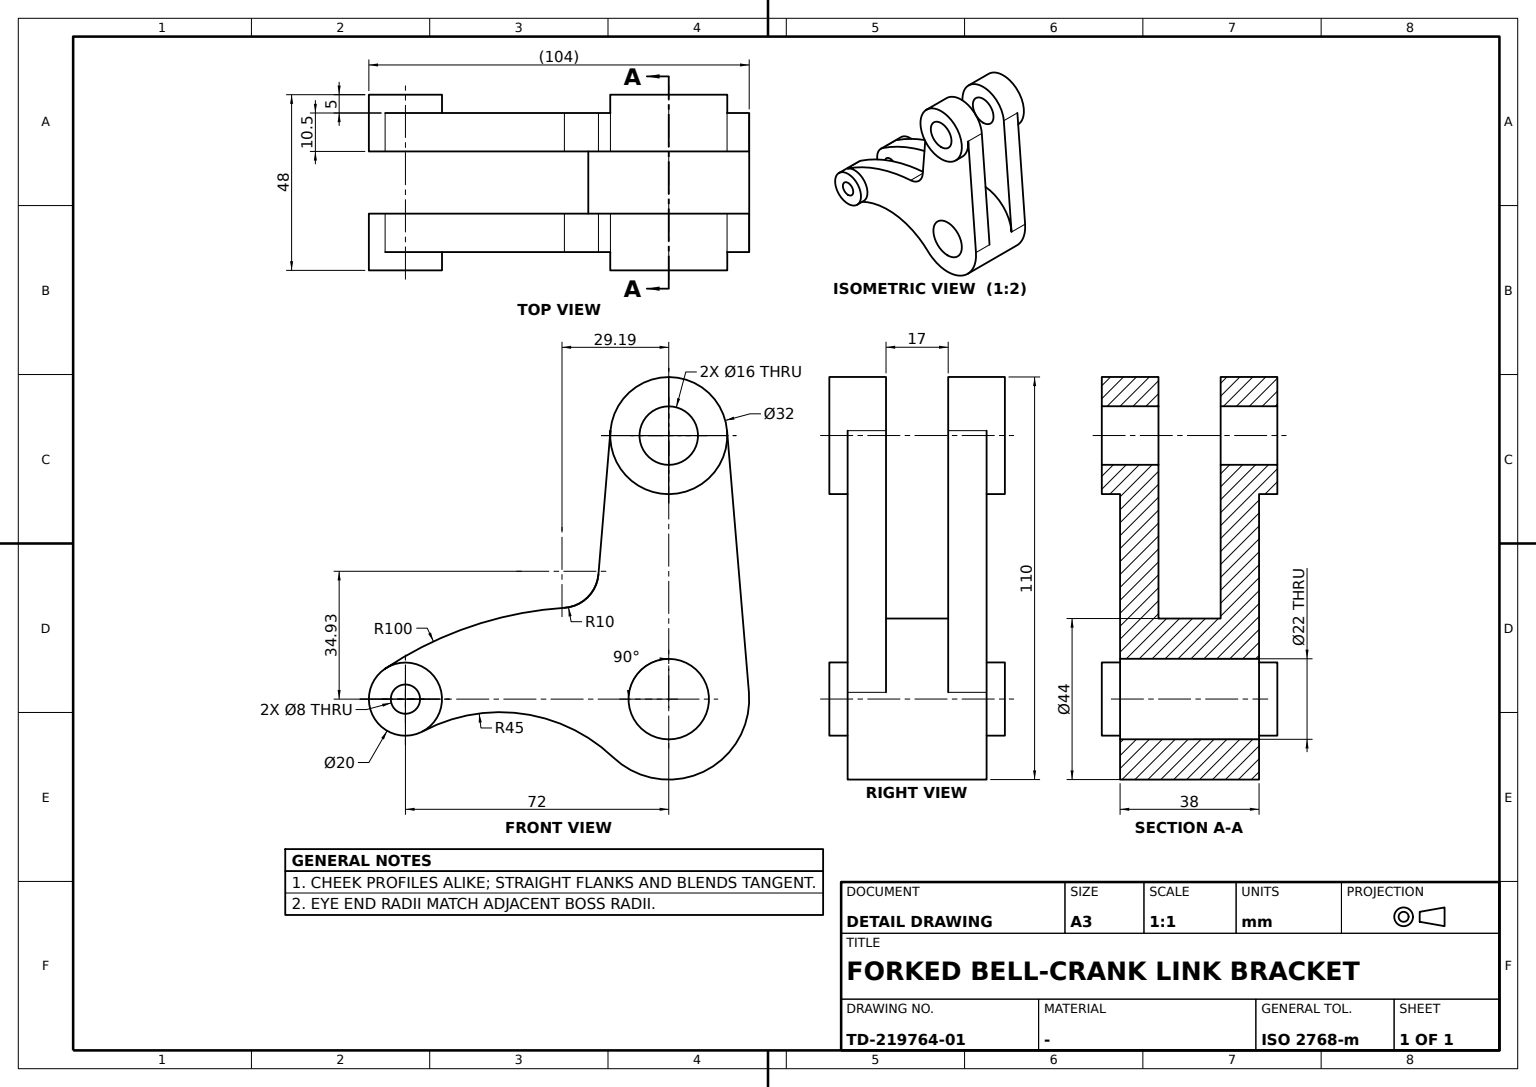
ISO-10303-21;
HEADER;
FILE_DESCRIPTION((''),'2;1');
FILE_NAME('','',(''),(''),'','','');
FILE_SCHEMA(('AUTOMOTIVE_DESIGN'));
ENDSEC;
DATA;
#1=APPLICATION_CONTEXT('');
#2=PRODUCT_CONTEXT('',#1,'mechanical');
#3=PRODUCT('','','',(#2));
#4=PRODUCT_DEFINITION_FORMATION('','',#3);
#5=PRODUCT_DEFINITION_CONTEXT('',#1,'design');
#6=PRODUCT_DEFINITION('','',#4,#5);
#7=PRODUCT_DEFINITION_SHAPE('','',#6);
#8=(LENGTH_UNIT()NAMED_UNIT(*)SI_UNIT(.MILLI.,.METRE.));
#9=(NAMED_UNIT(*)PLANE_ANGLE_UNIT()SI_UNIT($,.RADIAN.));
#10=(NAMED_UNIT(*)SI_UNIT($,.STERADIAN.)SOLID_ANGLE_UNIT());
#11=UNCERTAINTY_MEASURE_WITH_UNIT(LENGTH_MEASURE(0.005),#8,'distance_accuracy_value','');
#12=(GEOMETRIC_REPRESENTATION_CONTEXT(3)GLOBAL_UNCERTAINTY_ASSIGNED_CONTEXT((#11))GLOBAL_UNIT_ASSIGNED_CONTEXT((#8,#9,#10))REPRESENTATION_CONTEXT('',''));
#13=CARTESIAN_POINT('',(-24.,72.,-10.));
#14=VERTEX_POINT('',#13);
#15=CARTESIAN_POINT('',(-24.,72.,0.));
#16=DIRECTION('',(1.,0.,0.));
#17=DIRECTION('',(0.,0.,-1.));
#18=AXIS2_PLACEMENT_3D('',#15,#16,#17);
#19=CIRCLE('',#18,10.);
#20=EDGE_CURVE('',#14,#14,#19,.T.);
#21=ORIENTED_EDGE('',*,*,#20,.T.);
#22=EDGE_LOOP('',(#21));
#23=FACE_BOUND('',#22,.T.);
#24=CARTESIAN_POINT('',(-8.5,67.30303,-8.828277));
#25=VERTEX_POINT('',#24);
#26=CARTESIAN_POINT('',(-8.5,77.555257,8.314994));
#27=VERTEX_POINT('',#26);
#28=CARTESIAN_POINT('',(-8.5,72.,0.));
#29=AXIS2_PLACEMENT_3D('',#28,#16,#17);
#30=CIRCLE('',#29,10.);
#31=EDGE_CURVE('',#25,#27,#30,.T.);
#32=ORIENTED_EDGE('',*,*,#31,.F.);
#33=CARTESIAN_POINT('',(-19.,67.30303,-8.828277));
#34=VERTEX_POINT('',#33);
#35=CARTESIAN_POINT('',(-13.75,67.30303,-8.828277));
#36=VECTOR('',#16,1000.);
#37=LINE('',#35,#36);
#38=EDGE_CURVE('',#34,#25,#37,.T.);
#39=ORIENTED_EDGE('',*,*,#38,.F.);
#40=CARTESIAN_POINT('',(-19.,77.555257,8.314994));
#41=VERTEX_POINT('',#40);
#42=CARTESIAN_POINT('',(-19.,72.,0.));
#43=AXIS2_PLACEMENT_3D('',#42,#16,#17);
#44=CIRCLE('',#43,10.);
#45=EDGE_CURVE('',#41,#34,#44,.T.);
#46=ORIENTED_EDGE('',*,*,#45,.F.);
#47=CARTESIAN_POINT('',(-13.75,77.555257,8.314994));
#48=LINE('',#47,#36);
#49=EDGE_CURVE('',#41,#27,#48,.T.);
#50=ORIENTED_EDGE('',*,*,#49,.T.);
#51=EDGE_LOOP('',(#32,#39,#46,#50));
#52=FACE_BOUND('',#51,.T.);
#53=CARTESIAN_POINT('',(16.25,72.,0.));
#54=DIRECTION('',(0.,1.,0.));
#55=AXIS2_PLACEMENT_3D('',#53,#16,#54);
#56=CYLINDRICAL_SURFACE('',#55,10.);
#57=ADVANCED_FACE('',(#23,#52),#56,.T.);
#58=CARTESIAN_POINT('',(19.,67.30303,-8.828277));
#59=VERTEX_POINT('',#58);
#60=CARTESIAN_POINT('',(19.,15.159204,-15.943605));
#61=VERTEX_POINT('',#60);
#62=CARTESIAN_POINT('',(19.,46.166667,-48.555524));
#63=AXIS2_PLACEMENT_3D('',#62,#16,#17);
#64=CIRCLE('',#63,45.);
#65=EDGE_CURVE('',#59,#61,#64,.T.);
#66=ORIENTED_EDGE('',*,*,#65,.T.);
#67=CARTESIAN_POINT('',(8.5,15.159204,-15.943605));
#68=VERTEX_POINT('',#67);
#69=CARTESIAN_POINT('',(13.75,15.159204,-15.943605));
#70=LINE('',#69,#36);
#71=EDGE_CURVE('',#61,#68,#70,.F.);
#72=ORIENTED_EDGE('',*,*,#71,.T.);
#73=CARTESIAN_POINT('',(8.5,67.30303,-8.828277));
#74=VERTEX_POINT('',#73);
#75=CARTESIAN_POINT('',(8.5,46.166667,-48.555524));
#76=AXIS2_PLACEMENT_3D('',#75,#16,#17);
#77=CIRCLE('',#76,45.);
#78=EDGE_CURVE('',#74,#68,#77,.T.);
#79=ORIENTED_EDGE('',*,*,#78,.F.);
#80=CARTESIAN_POINT('',(13.75,67.30303,-8.828277));
#81=LINE('',#80,#36);
#82=EDGE_CURVE('',#59,#74,#81,.F.);
#83=ORIENTED_EDGE('',*,*,#82,.F.);
#84=EDGE_LOOP('',(#66,#72,#79,#83));
#85=FACE_BOUND('',#84,.T.);
#86=CARTESIAN_POINT('',(13.75,46.166667,-48.555524));
#87=AXIS2_PLACEMENT_3D('',#86,#16,#54);
#88=CYLINDRICAL_SURFACE('',#87,45.);
#89=ADVANCED_FACE('',(#85),#88,.F.);
#90=CARTESIAN_POINT('',(8.5,72.,-4.));
#91=VERTEX_POINT('',#90);
#92=CARTESIAN_POINT('',(8.5,72.,0.));
#93=AXIS2_PLACEMENT_3D('',#92,#16,#17);
#94=CIRCLE('',#93,4.);
#95=EDGE_CURVE('',#91,#91,#94,.T.);
#96=ORIENTED_EDGE('',*,*,#95,.T.);
#97=EDGE_LOOP('',(#96));
#98=FACE_BOUND('',#97,.T.);
#99=CARTESIAN_POINT('',(8.5,0.,64.));
#100=VERTEX_POINT('',#99);
#101=CARTESIAN_POINT('',(8.5,0.,72.));
#102=AXIS2_PLACEMENT_3D('',#101,#16,#17);
#103=CIRCLE('',#102,8.);
#104=EDGE_CURVE('',#100,#100,#103,.T.);
#105=ORIENTED_EDGE('',*,*,#104,.T.);
#106=EDGE_LOOP('',(#105));
#107=FACE_BOUND('',#106,.T.);
#108=ORIENTED_EDGE('',*,*,#78,.T.);
#109=CARTESIAN_POINT('',(8.5,-21.923478,1.833333));
#110=VERTEX_POINT('',#109);
#111=CARTESIAN_POINT('',(8.5,0.,0.));
#112=AXIS2_PLACEMENT_3D('',#111,#16,#17);
#113=CIRCLE('',#112,22.);
#114=EDGE_CURVE('',#68,#110,#113,.T.);
#115=ORIENTED_EDGE('',*,*,#114,.T.);
#116=CARTESIAN_POINT('',(8.5,-15.944348,73.333333));
#117=VERTEX_POINT('',#116);
#118=DIRECTION('',(0.,0.083333333,0.996521729));
#119=VECTOR('',#118,1000.);
#120=LINE('',#109,#119);
#121=EDGE_CURVE('',#110,#117,#120,.T.);
#122=ORIENTED_EDGE('',*,*,#121,.T.);
#123=CARTESIAN_POINT('',(8.5,15.944371,73.333051));
#124=VERTEX_POINT('',#123);
#125=CIRCLE('',#102,16.);
#126=EDGE_CURVE('',#124,#117,#125,.T.);
#127=ORIENTED_EDGE('',*,*,#126,.F.);
#128=CARTESIAN_POINT('',(8.5,19.224768,34.096843));
#129=VERTEX_POINT('',#128);
#130=DIRECTION('',(0.,0.083315682,-0.996523204));
#131=VECTOR('',#130,1000.);
#132=LINE('',#123,#131);
#133=EDGE_CURVE('',#124,#129,#132,.T.);
#134=ORIENTED_EDGE('',*,*,#133,.T.);
#135=CARTESIAN_POINT('',(8.5,28.536608,24.951369));
#136=VERTEX_POINT('',#135);
#137=CARTESIAN_POINT('',(8.5,29.19,34.93));
#138=AXIS2_PLACEMENT_3D('',#137,#16,#17);
#139=CIRCLE('',#138,10.);
#140=EDGE_CURVE('',#129,#136,#139,.T.);
#141=ORIENTED_EDGE('',*,*,#140,.T.);
#142=CARTESIAN_POINT('',(8.5,77.555257,8.314994));
#143=VERTEX_POINT('',#142);
#144=CARTESIAN_POINT('',(8.5,22.002686,-74.834942));
#145=AXIS2_PLACEMENT_3D('',#144,#16,#17);
#146=CIRCLE('',#145,100.);
#147=EDGE_CURVE('',#143,#136,#146,.T.);
#148=ORIENTED_EDGE('',*,*,#147,.F.);
#149=CIRCLE('',#93,10.);
#150=EDGE_CURVE('',#74,#143,#149,.T.);
#151=ORIENTED_EDGE('',*,*,#150,.F.);
#152=EDGE_LOOP('',(#108,#115,#122,#127,#134,#141,#148,#151));
#153=FACE_BOUND('',#152,.T.);
#154=AXIS2_PLACEMENT_3D('',#111,#16,#54);
#155=PLANE('',#154);
#156=ADVANCED_FACE('',(#98,#107,#153),#155,.F.);
#157=CARTESIAN_POINT('',(19.,28.536608,24.951369));
#158=VERTEX_POINT('',#157);
#159=CARTESIAN_POINT('',(13.75,28.536608,24.951369));
#160=LINE('',#159,#36);
#161=EDGE_CURVE('',#158,#136,#160,.F.);
#162=ORIENTED_EDGE('',*,*,#161,.F.);
#163=CARTESIAN_POINT('',(19.,77.555257,8.314994));
#164=VERTEX_POINT('',#163);
#165=CARTESIAN_POINT('',(19.,22.002686,-74.834942));
#166=AXIS2_PLACEMENT_3D('',#165,#16,#17);
#167=CIRCLE('',#166,100.);
#168=EDGE_CURVE('',#164,#158,#167,.T.);
#169=ORIENTED_EDGE('',*,*,#168,.F.);
#170=CARTESIAN_POINT('',(13.75,77.555257,8.314994));
#171=LINE('',#170,#36);
#172=EDGE_CURVE('',#164,#143,#171,.F.);
#173=ORIENTED_EDGE('',*,*,#172,.T.);
#174=ORIENTED_EDGE('',*,*,#147,.T.);
#175=EDGE_LOOP('',(#162,#169,#173,#174));
#176=FACE_BOUND('',#175,.T.);
#177=CARTESIAN_POINT('',(13.75,22.002686,-74.834942));
#178=AXIS2_PLACEMENT_3D('',#177,#16,#54);
#179=CYLINDRICAL_SURFACE('',#178,100.);
#180=ADVANCED_FACE('',(#176),#179,.T.);
#181=CARTESIAN_POINT('',(-19.,15.944371,73.333051));
#182=VERTEX_POINT('',#181);
#183=CARTESIAN_POINT('',(-19.,19.224768,34.096843));
#184=VERTEX_POINT('',#183);
#185=LINE('',#181,#131);
#186=EDGE_CURVE('',#182,#184,#185,.T.);
#187=ORIENTED_EDGE('',*,*,#186,.T.);
#188=CARTESIAN_POINT('',(-19.,28.536608,24.951369));
#189=VERTEX_POINT('',#188);
#190=CARTESIAN_POINT('',(-19.,29.19,34.93));
#191=AXIS2_PLACEMENT_3D('',#190,#16,#17);
#192=CIRCLE('',#191,10.);
#193=EDGE_CURVE('',#184,#189,#192,.T.);
#194=ORIENTED_EDGE('',*,*,#193,.T.);
#195=CARTESIAN_POINT('',(-19.,22.002686,-74.834942));
#196=AXIS2_PLACEMENT_3D('',#195,#16,#17);
#197=CIRCLE('',#196,100.);
#198=EDGE_CURVE('',#41,#189,#197,.T.);
#199=ORIENTED_EDGE('',*,*,#198,.F.);
#200=ORIENTED_EDGE('',*,*,#45,.T.);
#201=CARTESIAN_POINT('',(-19.,15.159204,-15.943605));
#202=VERTEX_POINT('',#201);
#203=CARTESIAN_POINT('',(-19.,46.166667,-48.555524));
#204=AXIS2_PLACEMENT_3D('',#203,#16,#17);
#205=CIRCLE('',#204,45.);
#206=EDGE_CURVE('',#34,#202,#205,.T.);
#207=ORIENTED_EDGE('',*,*,#206,.T.);
#208=CARTESIAN_POINT('',(-19.,-21.923478,1.833333));
#209=VERTEX_POINT('',#208);
#210=CARTESIAN_POINT('',(-19.,0.,0.));
#211=AXIS2_PLACEMENT_3D('',#210,#16,#17);
#212=CIRCLE('',#211,22.);
#213=EDGE_CURVE('',#209,#202,#212,.T.);
#214=ORIENTED_EDGE('',*,*,#213,.F.);
#215=CARTESIAN_POINT('',(-19.,-15.944348,73.333333));
#216=VERTEX_POINT('',#215);
#217=LINE('',#208,#119);
#218=EDGE_CURVE('',#209,#216,#217,.T.);
#219=ORIENTED_EDGE('',*,*,#218,.T.);
#220=CARTESIAN_POINT('',(-19.,0.,72.));
#221=AXIS2_PLACEMENT_3D('',#220,#16,#17);
#222=CIRCLE('',#221,16.);
#223=EDGE_CURVE('',#216,#182,#222,.T.);
#224=ORIENTED_EDGE('',*,*,#223,.T.);
#225=EDGE_LOOP('',(#187,#194,#199,#200,#207,#214,#219,#224));
#226=FACE_BOUND('',#225,.T.);
#227=CARTESIAN_POINT('',(-19.,0.,-11.));
#228=VERTEX_POINT('',#227);
#229=CIRCLE('',#211,11.);
#230=EDGE_CURVE('',#228,#228,#229,.T.);
#231=ORIENTED_EDGE('',*,*,#230,.T.);
#232=EDGE_LOOP('',(#231));
#233=FACE_BOUND('',#232,.T.);
#234=AXIS2_PLACEMENT_3D('',#210,#16,#54);
#235=PLANE('',#234);
#236=ADVANCED_FACE('',(#226,#233),#235,.F.);
#237=CARTESIAN_POINT('',(19.,-21.923478,1.833333));
#238=VERTEX_POINT('',#237);
#239=CARTESIAN_POINT('',(19.,-15.944348,73.333333));
#240=VERTEX_POINT('',#239);
#241=LINE('',#237,#119);
#242=EDGE_CURVE('',#238,#240,#241,.T.);
#243=ORIENTED_EDGE('',*,*,#242,.T.);
#244=CARTESIAN_POINT('',(16.25,-15.944348,73.333333));
#245=LINE('',#244,#36);
#246=EDGE_CURVE('',#117,#240,#245,.T.);
#247=ORIENTED_EDGE('',*,*,#246,.F.);
#248=ORIENTED_EDGE('',*,*,#121,.F.);
#249=CARTESIAN_POINT('',(0.,-21.923478,1.833333));
#250=LINE('',#249,#36);
#251=EDGE_CURVE('',#238,#110,#250,.F.);
#252=ORIENTED_EDGE('',*,*,#251,.F.);
#253=EDGE_LOOP('',(#243,#247,#248,#252));
#254=FACE_BOUND('',#253,.T.);
#255=DIRECTION('',(0.,-0.996521729,0.083333333));
#256=AXIS2_PLACEMENT_3D('',#237,#255,#118);
#257=PLANE('',#256);
#258=ADVANCED_FACE('',(#254),#257,.T.);
#259=CARTESIAN_POINT('',(-8.5,15.944371,73.333051));
#260=VERTEX_POINT('',#259);
#261=CARTESIAN_POINT('',(16.25,15.944371,73.333051));
#262=LINE('',#261,#36);
#263=EDGE_CURVE('',#260,#182,#262,.F.);
#264=ORIENTED_EDGE('',*,*,#263,.T.);
#265=ORIENTED_EDGE('',*,*,#223,.F.);
#266=CARTESIAN_POINT('',(-8.5,-15.944348,73.333333));
#267=VERTEX_POINT('',#266);
#268=EDGE_CURVE('',#267,#216,#245,.F.);
#269=ORIENTED_EDGE('',*,*,#268,.F.);
#270=CARTESIAN_POINT('',(-8.5,0.,72.));
#271=AXIS2_PLACEMENT_3D('',#270,#16,#17);
#272=CIRCLE('',#271,16.);
#273=EDGE_CURVE('',#260,#267,#272,.T.);
#274=ORIENTED_EDGE('',*,*,#273,.F.);
#275=EDGE_LOOP('',(#264,#265,#269,#274));
#276=FACE_BOUND('',#275,.T.);
#277=CARTESIAN_POINT('',(-24.,0.,56.));
#278=VERTEX_POINT('',#277);
#279=CARTESIAN_POINT('',(-24.,0.,72.));
#280=AXIS2_PLACEMENT_3D('',#279,#16,#17);
#281=CIRCLE('',#280,16.);
#282=EDGE_CURVE('',#278,#278,#281,.T.);
#283=ORIENTED_EDGE('',*,*,#282,.T.);
#284=EDGE_LOOP('',(#283));
#285=FACE_BOUND('',#284,.T.);
#286=CARTESIAN_POINT('',(16.25,0.,72.));
#287=AXIS2_PLACEMENT_3D('',#286,#16,#54);
#288=CYLINDRICAL_SURFACE('',#287,16.);
#289=ADVANCED_FACE('',(#276,#285),#288,.T.);
#290=CARTESIAN_POINT('',(-8.5,15.159204,-15.943605));
#291=VERTEX_POINT('',#290);
#292=CARTESIAN_POINT('',(-8.5,-21.923478,1.833333));
#293=VERTEX_POINT('',#292);
#294=CARTESIAN_POINT('',(-8.5,0.,0.));
#295=AXIS2_PLACEMENT_3D('',#294,#16,#17);
#296=CIRCLE('',#295,22.);
#297=EDGE_CURVE('',#291,#293,#296,.T.);
#298=ORIENTED_EDGE('',*,*,#297,.T.);
#299=EDGE_CURVE('',#209,#293,#250,.T.);
#300=ORIENTED_EDGE('',*,*,#299,.F.);
#301=ORIENTED_EDGE('',*,*,#213,.T.);
#302=CARTESIAN_POINT('',(-13.75,15.159204,-15.943605));
#303=LINE('',#302,#36);
#304=EDGE_CURVE('',#202,#291,#303,.T.);
#305=ORIENTED_EDGE('',*,*,#304,.T.);
#306=EDGE_LOOP('',(#298,#300,#301,#305));
#307=FACE_BOUND('',#306,.T.);
#308=ORIENTED_EDGE('',*,*,#71,.F.);
#309=CARTESIAN_POINT('',(19.,0.,0.));
#310=AXIS2_PLACEMENT_3D('',#309,#16,#17);
#311=CIRCLE('',#310,22.);
#312=EDGE_CURVE('',#238,#61,#311,.T.);
#313=ORIENTED_EDGE('',*,*,#312,.F.);
#314=ORIENTED_EDGE('',*,*,#251,.T.);
#315=ORIENTED_EDGE('',*,*,#114,.F.);
#316=EDGE_LOOP('',(#308,#313,#314,#315));
#317=FACE_BOUND('',#316,.T.);
#318=CARTESIAN_POINT('',(0.,0.,0.));
#319=AXIS2_PLACEMENT_3D('',#318,#16,#54);
#320=CYLINDRICAL_SURFACE('',#319,22.);
#321=ADVANCED_FACE('',(#307,#317),#320,.T.);
#322=CARTESIAN_POINT('',(-8.5,46.166667,-48.555524));
#323=AXIS2_PLACEMENT_3D('',#322,#16,#17);
#324=CIRCLE('',#323,45.);
#325=EDGE_CURVE('',#25,#291,#324,.T.);
#326=ORIENTED_EDGE('',*,*,#325,.T.);
#327=ORIENTED_EDGE('',*,*,#304,.F.);
#328=ORIENTED_EDGE('',*,*,#206,.F.);
#329=ORIENTED_EDGE('',*,*,#38,.T.);
#330=EDGE_LOOP('',(#326,#327,#328,#329));
#331=FACE_BOUND('',#330,.T.);
#332=ADVANCED_FACE('',(#331),#88,.F.);
#333=CARTESIAN_POINT('',(-24.,0.,64.));
#334=VERTEX_POINT('',#333);
#335=CIRCLE('',#280,8.);
#336=EDGE_CURVE('',#334,#334,#335,.T.);
#337=ORIENTED_EDGE('',*,*,#336,.F.);
#338=EDGE_LOOP('',(#337));
#339=FACE_BOUND('',#338,.T.);
#340=CARTESIAN_POINT('',(-8.5,0.,64.));
#341=VERTEX_POINT('',#340);
#342=CIRCLE('',#271,8.);
#343=EDGE_CURVE('',#341,#341,#342,.T.);
#344=ORIENTED_EDGE('',*,*,#343,.T.);
#345=EDGE_LOOP('',(#344));
#346=FACE_BOUND('',#345,.T.);
#347=CYLINDRICAL_SURFACE('',#287,8.);
#348=ADVANCED_FACE('',(#339,#346),#347,.F.);
#349=CARTESIAN_POINT('',(-8.5,19.224768,34.096843));
#350=VERTEX_POINT('',#349);
#351=CARTESIAN_POINT('',(13.75,19.224768,34.096843));
#352=LINE('',#351,#36);
#353=EDGE_CURVE('',#184,#350,#352,.T.);
#354=ORIENTED_EDGE('',*,*,#353,.F.);
#355=ORIENTED_EDGE('',*,*,#186,.F.);
#356=ORIENTED_EDGE('',*,*,#263,.F.);
#357=LINE('',#259,#131);
#358=EDGE_CURVE('',#260,#350,#357,.T.);
#359=ORIENTED_EDGE('',*,*,#358,.T.);
#360=EDGE_LOOP('',(#354,#355,#356,#359));
#361=FACE_BOUND('',#360,.T.);
#362=CARTESIAN_POINT('',(19.,15.944371,73.333051));
#363=DIRECTION('',(0.,0.996523204,0.083315682));
#364=AXIS2_PLACEMENT_3D('',#362,#363,#130);
#365=PLANE('',#364);
#366=ADVANCED_FACE('',(#361),#365,.T.);
#367=CARTESIAN_POINT('',(24.,72.,-4.));
#368=VERTEX_POINT('',#367);
#369=CARTESIAN_POINT('',(24.,72.,0.));
#370=AXIS2_PLACEMENT_3D('',#369,#16,#17);
#371=CIRCLE('',#370,4.);
#372=EDGE_CURVE('',#368,#368,#371,.T.);
#373=ORIENTED_EDGE('',*,*,#372,.T.);
#374=EDGE_LOOP('',(#373));
#375=FACE_BOUND('',#374,.T.);
#376=ORIENTED_EDGE('',*,*,#95,.F.);
#377=EDGE_LOOP('',(#376));
#378=FACE_BOUND('',#377,.T.);
#379=CYLINDRICAL_SURFACE('',#55,4.);
#380=ADVANCED_FACE('',(#375,#378),#379,.F.);
#381=ORIENTED_EDGE('',*,*,#372,.F.);
#382=EDGE_LOOP('',(#381));
#383=FACE_BOUND('',#382,.T.);
#384=CARTESIAN_POINT('',(24.,72.,-10.));
#385=VERTEX_POINT('',#384);
#386=CIRCLE('',#370,10.);
#387=EDGE_CURVE('',#385,#385,#386,.T.);
#388=ORIENTED_EDGE('',*,*,#387,.T.);
#389=EDGE_LOOP('',(#388));
#390=FACE_BOUND('',#389,.T.);
#391=CARTESIAN_POINT('',(24.,0.,0.));
#392=AXIS2_PLACEMENT_3D('',#391,#16,#54);
#393=PLANE('',#392);
#394=ADVANCED_FACE('',(#383,#390),#393,.T.);
#395=CARTESIAN_POINT('',(-8.5,28.536608,24.951369));
#396=VERTEX_POINT('',#395);
#397=CARTESIAN_POINT('',(-8.5,22.002686,-74.834942));
#398=AXIS2_PLACEMENT_3D('',#397,#16,#17);
#399=CIRCLE('',#398,100.);
#400=EDGE_CURVE('',#27,#396,#399,.T.);
#401=ORIENTED_EDGE('',*,*,#400,.F.);
#402=ORIENTED_EDGE('',*,*,#49,.F.);
#403=ORIENTED_EDGE('',*,*,#198,.T.);
#404=CARTESIAN_POINT('',(-13.75,28.536608,24.951369));
#405=LINE('',#404,#36);
#406=EDGE_CURVE('',#189,#396,#405,.T.);
#407=ORIENTED_EDGE('',*,*,#406,.T.);
#408=EDGE_LOOP('',(#401,#402,#403,#407));
#409=FACE_BOUND('',#408,.T.);
#410=ADVANCED_FACE('',(#409),#179,.T.);
#411=ORIENTED_EDGE('',*,*,#161,.T.);
#412=ORIENTED_EDGE('',*,*,#140,.F.);
#413=CARTESIAN_POINT('',(19.,19.224768,34.096843));
#414=VERTEX_POINT('',#413);
#415=EDGE_CURVE('',#414,#129,#352,.F.);
#416=ORIENTED_EDGE('',*,*,#415,.F.);
#417=CARTESIAN_POINT('',(19.,29.19,34.93));
#418=AXIS2_PLACEMENT_3D('',#417,#16,#17);
#419=CIRCLE('',#418,10.);
#420=EDGE_CURVE('',#414,#158,#419,.T.);
#421=ORIENTED_EDGE('',*,*,#420,.T.);
#422=EDGE_LOOP('',(#411,#412,#416,#421));
#423=FACE_BOUND('',#422,.T.);
#424=CARTESIAN_POINT('',(13.75,29.19,34.93));
#425=AXIS2_PLACEMENT_3D('',#424,#16,#54);
#426=CYLINDRICAL_SURFACE('',#425,10.);
#427=ADVANCED_FACE('',(#423),#426,.F.);
#428=ORIENTED_EDGE('',*,*,#230,.F.);
#429=EDGE_LOOP('',(#428));
#430=FACE_BOUND('',#429,.T.);
#431=CARTESIAN_POINT('',(19.,0.,-11.));
#432=VERTEX_POINT('',#431);
#433=CIRCLE('',#310,11.);
#434=EDGE_CURVE('',#432,#432,#433,.T.);
#435=ORIENTED_EDGE('',*,*,#434,.T.);
#436=EDGE_LOOP('',(#435));
#437=FACE_BOUND('',#436,.T.);
#438=CYLINDRICAL_SURFACE('',#319,11.);
#439=ADVANCED_FACE('',(#430,#437),#438,.F.);
#440=CARTESIAN_POINT('',(24.,0.,64.));
#441=VERTEX_POINT('',#440);
#442=CARTESIAN_POINT('',(24.,0.,72.));
#443=AXIS2_PLACEMENT_3D('',#442,#16,#17);
#444=CIRCLE('',#443,8.);
#445=EDGE_CURVE('',#441,#441,#444,.T.);
#446=ORIENTED_EDGE('',*,*,#445,.T.);
#447=EDGE_LOOP('',(#446));
#448=FACE_BOUND('',#447,.T.);
#449=ORIENTED_EDGE('',*,*,#104,.F.);
#450=EDGE_LOOP('',(#449));
#451=FACE_BOUND('',#450,.T.);
#452=ADVANCED_FACE('',(#448,#451),#347,.F.);
#453=ORIENTED_EDGE('',*,*,#126,.T.);
#454=ORIENTED_EDGE('',*,*,#246,.T.);
#455=VERTEX_POINT('',#362);
#456=CARTESIAN_POINT('',(19.,0.,72.));
#457=AXIS2_PLACEMENT_3D('',#456,#16,#17);
#458=CIRCLE('',#457,16.);
#459=EDGE_CURVE('',#240,#455,#458,.T.);
#460=ORIENTED_EDGE('',*,*,#459,.T.);
#461=EDGE_CURVE('',#124,#455,#262,.T.);
#462=ORIENTED_EDGE('',*,*,#461,.F.);
#463=EDGE_LOOP('',(#453,#454,#460,#462));
#464=FACE_BOUND('',#463,.T.);
#465=CARTESIAN_POINT('',(24.,0.,56.));
#466=VERTEX_POINT('',#465);
#467=CIRCLE('',#443,16.);
#468=EDGE_CURVE('',#466,#466,#467,.T.);
#469=ORIENTED_EDGE('',*,*,#468,.F.);
#470=EDGE_LOOP('',(#469));
#471=FACE_BOUND('',#470,.T.);
#472=ADVANCED_FACE('',(#464,#471),#288,.T.);
#473=ORIENTED_EDGE('',*,*,#268,.T.);
#474=ORIENTED_EDGE('',*,*,#218,.F.);
#475=ORIENTED_EDGE('',*,*,#299,.T.);
#476=LINE('',#292,#119);
#477=EDGE_CURVE('',#293,#267,#476,.T.);
#478=ORIENTED_EDGE('',*,*,#477,.T.);
#479=EDGE_LOOP('',(#473,#474,#475,#478));
#480=FACE_BOUND('',#479,.T.);
#481=ADVANCED_FACE('',(#480),#257,.T.);
#482=ORIENTED_EDGE('',*,*,#434,.F.);
#483=EDGE_LOOP('',(#482));
#484=FACE_BOUND('',#483,.T.);
#485=ORIENTED_EDGE('',*,*,#65,.F.);
#486=CARTESIAN_POINT('',(19.,72.,0.));
#487=AXIS2_PLACEMENT_3D('',#486,#16,#17);
#488=CIRCLE('',#487,10.);
#489=EDGE_CURVE('',#164,#59,#488,.T.);
#490=ORIENTED_EDGE('',*,*,#489,.F.);
#491=ORIENTED_EDGE('',*,*,#168,.T.);
#492=ORIENTED_EDGE('',*,*,#420,.F.);
#493=LINE('',#362,#131);
#494=EDGE_CURVE('',#455,#414,#493,.T.);
#495=ORIENTED_EDGE('',*,*,#494,.F.);
#496=ORIENTED_EDGE('',*,*,#459,.F.);
#497=ORIENTED_EDGE('',*,*,#242,.F.);
#498=ORIENTED_EDGE('',*,*,#312,.T.);
#499=EDGE_LOOP('',(#485,#490,#491,#492,#495,#496,#497,#498));
#500=FACE_BOUND('',#499,.T.);
#501=AXIS2_PLACEMENT_3D('',#309,#16,#54);
#502=PLANE('',#501);
#503=ADVANCED_FACE('',(#484,#500),#502,.T.);
#504=ORIENTED_EDGE('',*,*,#133,.F.);
#505=ORIENTED_EDGE('',*,*,#461,.T.);
#506=ORIENTED_EDGE('',*,*,#494,.T.);
#507=ORIENTED_EDGE('',*,*,#415,.T.);
#508=EDGE_LOOP('',(#504,#505,#506,#507));
#509=FACE_BOUND('',#508,.T.);
#510=ADVANCED_FACE('',(#509),#365,.T.);
#511=ORIENTED_EDGE('',*,*,#406,.F.);
#512=ORIENTED_EDGE('',*,*,#193,.F.);
#513=ORIENTED_EDGE('',*,*,#353,.T.);
#514=CARTESIAN_POINT('',(-8.5,29.19,34.93));
#515=AXIS2_PLACEMENT_3D('',#514,#16,#17);
#516=CIRCLE('',#515,10.);
#517=EDGE_CURVE('',#350,#396,#516,.T.);
#518=ORIENTED_EDGE('',*,*,#517,.T.);
#519=EDGE_LOOP('',(#511,#512,#513,#518));
#520=FACE_BOUND('',#519,.T.);
#521=ADVANCED_FACE('',(#520),#426,.F.);
#522=CARTESIAN_POINT('',(-8.5,72.,-4.));
#523=VERTEX_POINT('',#522);
#524=CIRCLE('',#29,4.);
#525=EDGE_CURVE('',#523,#523,#524,.T.);
#526=ORIENTED_EDGE('',*,*,#525,.F.);
#527=EDGE_LOOP('',(#526));
#528=FACE_BOUND('',#527,.T.);
#529=ORIENTED_EDGE('',*,*,#273,.T.);
#530=ORIENTED_EDGE('',*,*,#477,.F.);
#531=ORIENTED_EDGE('',*,*,#297,.F.);
#532=ORIENTED_EDGE('',*,*,#325,.F.);
#533=ORIENTED_EDGE('',*,*,#31,.T.);
#534=ORIENTED_EDGE('',*,*,#400,.T.);
#535=ORIENTED_EDGE('',*,*,#517,.F.);
#536=ORIENTED_EDGE('',*,*,#358,.F.);
#537=EDGE_LOOP('',(#529,#530,#531,#532,#533,#534,#535,#536));
#538=FACE_BOUND('',#537,.T.);
#539=ORIENTED_EDGE('',*,*,#343,.F.);
#540=EDGE_LOOP('',(#539));
#541=FACE_BOUND('',#540,.T.);
#542=AXIS2_PLACEMENT_3D('',#294,#16,#54);
#543=PLANE('',#542);
#544=ADVANCED_FACE('',(#528,#538,#541),#543,.T.);
#545=ORIENTED_EDGE('',*,*,#336,.T.);
#546=EDGE_LOOP('',(#545));
#547=FACE_BOUND('',#546,.T.);
#548=ORIENTED_EDGE('',*,*,#282,.F.);
#549=EDGE_LOOP('',(#548));
#550=FACE_BOUND('',#549,.T.);
#551=CARTESIAN_POINT('',(-24.,0.,0.));
#552=AXIS2_PLACEMENT_3D('',#551,#16,#54);
#553=PLANE('',#552);
#554=ADVANCED_FACE('',(#547,#550),#553,.F.);
#555=ORIENTED_EDGE('',*,*,#525,.T.);
#556=EDGE_LOOP('',(#555));
#557=FACE_BOUND('',#556,.T.);
#558=CARTESIAN_POINT('',(-24.,72.,-4.));
#559=VERTEX_POINT('',#558);
#560=CIRCLE('',#18,4.);
#561=EDGE_CURVE('',#559,#559,#560,.T.);
#562=ORIENTED_EDGE('',*,*,#561,.F.);
#563=EDGE_LOOP('',(#562));
#564=FACE_BOUND('',#563,.T.);
#565=ADVANCED_FACE('',(#557,#564),#379,.F.);
#566=ORIENTED_EDGE('',*,*,#387,.F.);
#567=EDGE_LOOP('',(#566));
#568=FACE_BOUND('',#567,.T.);
#569=ORIENTED_EDGE('',*,*,#489,.T.);
#570=ORIENTED_EDGE('',*,*,#82,.T.);
#571=ORIENTED_EDGE('',*,*,#150,.T.);
#572=ORIENTED_EDGE('',*,*,#172,.F.);
#573=EDGE_LOOP('',(#569,#570,#571,#572));
#574=FACE_BOUND('',#573,.T.);
#575=ADVANCED_FACE('',(#568,#574),#56,.T.);
#576=ORIENTED_EDGE('',*,*,#468,.T.);
#577=EDGE_LOOP('',(#576));
#578=FACE_BOUND('',#577,.T.);
#579=ORIENTED_EDGE('',*,*,#445,.F.);
#580=EDGE_LOOP('',(#579));
#581=FACE_BOUND('',#580,.T.);
#582=ADVANCED_FACE('',(#578,#581),#393,.T.);
#583=ORIENTED_EDGE('',*,*,#561,.T.);
#584=EDGE_LOOP('',(#583));
#585=FACE_BOUND('',#584,.T.);
#586=ORIENTED_EDGE('',*,*,#20,.F.);
#587=EDGE_LOOP('',(#586));
#588=FACE_BOUND('',#587,.T.);
#589=ADVANCED_FACE('',(#585,#588),#553,.F.);
#590=CLOSED_SHELL('',(#57,#89,#156,#180,#236,#258,#289,#321,#332,#348,#366,#380,#394,#410,#427,#439,#452,#472,#481,#503,#510,#521,#544,#554,#565,#575,#582,#589));
#591=MANIFOLD_SOLID_BREP('',#590);
#592=ADVANCED_BREP_SHAPE_REPRESENTATION('',(#591),#12);
#593=SHAPE_DEFINITION_REPRESENTATION(#7,#592);
ENDSEC;
END-ISO-10303-21;
